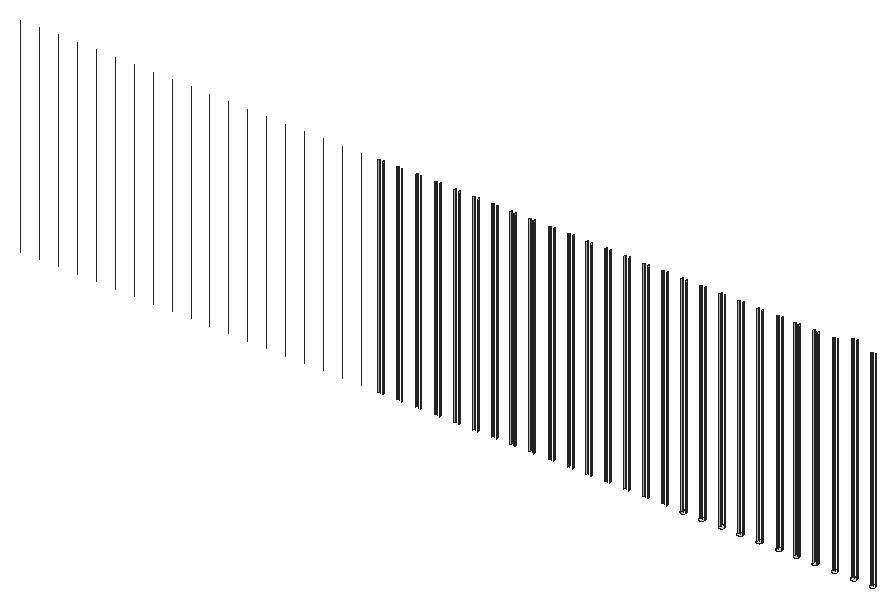
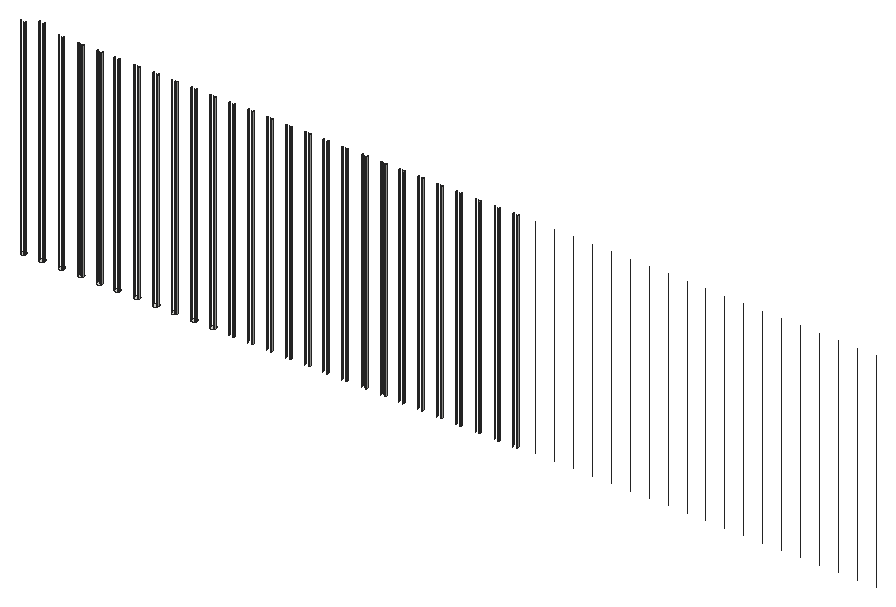
# SketchUp Ruby script. Lengths in inches.
U = 1.inch
M = Sketchup.active_model
def pt(a) = Geom::Point3d.new(a.map { |v| v * U })
def face(e, loops, mat)
  f = e.add_face(loops[0].map { |a| pt(a) })
  loops[1..].each { |l| e.add_face(l.map { |a| pt(a) }).erase! }
  f.material = f.back_material = mat if mat
  f
end
# faces: each face lists its corners as indices into pts; further lists are holes
def faces(e, pts, list, mat = nil) = list.each { |f| face(e, (f[0].is_a?(Array) ? f : [f]).map { |l| l.map { |i| pts[i] } }, mat) }
# xy, xz, yz: faces in a plane at the given z, y or x. An outline is a flat list of corners, or four numbers for a rectangle; further outlines are holes
def ring(l) = l.size == 4 ? [[l[0], l[1]], [l[2], l[1]], [l[2], l[3]], [l[0], l[3]]] : l.each_slice(2).to_a
def flat(e, list, mat, &to3) = list.each { |f| face(e, (f[0].is_a?(Array) ? f : [f]).map { |l| ring(l).map { |u, v| to3.(u, v) } }, mat) }
def xy(e, z, list, mat = nil) = flat(e, list, mat) { |x, y| [x, y, z] }
def xz(e, y, list, mat = nil) = flat(e, list, mat) { |x, z| [x, y, z] }
def yz(e, x, list, mat = nil) = flat(e, list, mat) { |y, z| [x, y, z] }
def lines(e, pts, list) = list.each { |a, b| e.add_line(pt(pts[a]), pt(pts[b])) }
# prism: a flat outline (further loops are holes) pulled along v
def prism(e, loops, v, mat = nil)
  f = face(e, loops, mat); d = Geom::Vector3d.new(v.map { |x| x * U })
  f.pushpull(f.normal.samedirection?(d) ? d.length : -d.length)
end
def box(e, o, s, mat = nil) = prism(e, [[o, [o[0] + s[0], o[1], o[2]], [o[0] + s[0], o[1] + s[1], o[2]], [o[0], o[1] + s[1], o[2]]]], [0, 0, s[2]], mat)
def at(x, y, z, deg = 0) = Geom::Transformation.translation(pt([x, y, z])) * Geom::Transformation.rotation(ORIGIN, Z_AXIS, deg.degrees)
def axes(o, x, y, z) = Geom::Transformation.new([*x, 0, *y, 0, *z, 0, *pt(o).to_a, 1])
def part(name) = M.definitions.add(name)
# library, detail: a bought-in or finely detailed component or shape, given as its bounding box
def library(name, o, s) = part(name).tap { |d| box(d.entities, o, s) }
def detail(e, o, s) = box(e.add_group.entities, o, s)
def put(e, d, t, mat = nil) = e.add_instance(d, t).tap { |i| i.material = mat if mat }
def group(e, t, mat = nil) = e.add_group.tap { |g| g.transformation = t; g.material = mat if mat }.entities
root = M.entities
xy(root,819.75,[[459.95,127.81,459.74,127.83,459.54,127.91,459.375,128.04,459.24,128.21,459.16,128.41,459.14,128.62,459.16,128.83,459.24,129.02,459.375,129.19,459.54,129.32,459.74,129.4,459.95,129.43,460.16,129.4,460.35,129.32,460.52,129.19,460.65,129.02,460.73,128.83,460.76,128.62,460.73,128.41,460.65,128.21,460.52,128.04,460.35,127.91,460.16,127.83],[465.76,127.81,465.55,127.83,465.35,127.91,465.1875,128.04,465.06,128.21,464.98,128.41,464.95,128.62,464.98,128.83,465.06,129.02,465.1875,129.19,465.35,129.32,465.55,129.4,465.76,129.43,465.97,129.4,466.17,129.32,466.34,129.19,466.46,129.02,466.55,128.83,466.57,128.62,466.55,128.41,466.46,128.21,466.34,128.04,466.17,127.91,465.97,127.83],[471.95,127.81,471.74,127.83,471.54,127.91,471.375,128.04,471.24,128.21,471.16,128.41,471.14,128.62,471.16,128.83,471.24,129.02,471.375,129.19,471.54,129.32,471.74,129.4,471.95,129.43,472.16,129.4,472.35,129.32,472.52,129.19,472.65,129.02,472.73,128.83,472.76,128.62,472.73,128.41,472.65,128.21,472.52,128.04,472.35,127.91,472.16,127.83],[477.76,127.81,477.55,127.83,477.35,127.91,477.1875,128.04,477.06,128.21,476.98,128.41,476.95,128.62,476.98,128.83,477.06,129.02,477.1875,129.19,477.35,129.32,477.55,129.4,477.76,129.43,477.97,129.4,478.17,129.32,478.34,129.19,478.46,129.02,478.55,128.83,478.57,128.62,478.55,128.41,478.46,128.21,478.34,128.04,478.17,127.91,477.97,127.83],[483.76,127.81,483.55,127.83,483.35,127.91,483.1875,128.04,483.06,128.21,482.98,128.41,482.95,128.62,482.98,128.83,483.06,129.02,483.1875,129.19,483.35,129.32,483.55,129.4,483.76,129.43,483.97,129.4,484.17,129.32,484.34,129.19,484.46,129.02,484.55,128.83,484.57,128.62,484.55,128.41,484.46,128.21,484.34,128.04,484.17,127.91,483.97,127.83],
  [489.89,127.81,489.68,127.83,489.48,127.91,489.3125,128.04,489.18,128.21,489.1,128.41,489.07,128.62,489.1,128.83,489.18,129.02,489.3125,129.19,489.48,129.32,489.68,129.4,489.89,129.43,490.1,129.4,490.29,129.32,490.46,129.19,490.59,129.02,490.67,128.83,490.7,128.62,490.67,128.41,490.59,128.21,490.46,128.04,490.29,127.91,490.1,127.83],[495.39,127.81,495.18,127.83,494.98,127.91,494.8125,128.04,494.68,128.21,494.6,128.41,494.57,128.62,494.6,128.83,494.68,129.02,494.8125,129.19,494.98,129.32,495.18,129.4,495.39,129.43,495.6,129.4,495.79,129.32,495.96,129.19,496.09,129.02,496.17,128.83,496.2,128.62,496.17,128.41,496.09,128.21,495.96,128.04,495.79,127.91,495.6,127.83],[501.32,127.81,501.11,127.83,500.92,127.91,500.75,128.04,500.62,128.21,500.54,128.41,500.51,128.62,500.54,128.83,500.62,129.02,500.75,129.19,500.92,129.32,501.11,129.4,501.32,129.43,501.53,129.4,501.73,129.32,501.9,129.19,502.03,129.02,502.11,128.83,502.14,128.62,502.11,128.41,502.03,128.21,501.9,128.04,501.73,127.91,501.53,127.83],[507.39,127.81,507.18,127.83,506.98,127.91,506.8125,128.04,506.68,128.21,506.6,128.41,506.57,128.62,506.6,128.83,506.68,129.02,506.8125,129.19,506.98,129.32,507.18,129.4,507.39,129.43,507.6,129.4,507.79,129.32,507.96,129.19,508.09,129.02,508.17,128.83,508.2,128.62,508.17,128.41,508.09,128.21,507.96,128.04,507.79,127.91,507.6,127.83],[513.45,127.81,513.24,127.83,513.04,127.91,512.875,128.04,512.74,128.21,512.66,128.41,512.64,128.62,512.66,128.83,512.74,129.02,512.875,129.19,513.04,129.32,513.24,129.4,513.45,129.43,513.66,129.4,513.85,129.32,514.02,129.19,514.15,129.02,514.23,128.83,514.26,128.62,514.23,128.41,514.15,128.21,514.02,128.04,513.85,127.91,513.66,127.83],
  [519.32,127.81,519.11,127.83,518.92,127.91,518.75,128.04,518.62,128.21,518.54,128.41,518.51,128.62,518.54,128.83,518.62,129.02,518.75,129.19,518.92,129.32,519.11,129.4,519.32,129.43,519.53,129.4,519.73,129.32,519.9,129.19,520.03,129.02,520.11,128.83,520.14,128.62,520.11,128.41,520.03,128.21,519.9,128.04,519.73,127.91,519.53,127.83]])
p = [[364.23,128.83,819.75],[364.2,128.62,819.75],[364.2,128.62,884.89],[364.23,128.83,884.89],[365.82,128.62,819.75],[365.8,128.83,819.75],
  [365.8,128.83,884.89],[365.82,128.62,884.89],[369.98,128.83,819.75],[369.95,128.62,819.75],[369.95,128.62,884.89],[369.98,128.83,884.89],
  [371.57,128.62,819.75],[371.55,128.83,819.75],[371.55,128.83,884.89],[371.57,128.62,884.89],[375.91,128.83,819.75],[375.89,128.62,819.75],
  [375.89,128.62,884.89],[375.91,128.83,884.89],[377.51,128.62,819.75],[377.48,128.83,819.75],[377.48,128.83,884.89],[377.51,128.62,884.89],
  [381.98,128.83,819.75],[381.95,128.62,819.75],[381.95,128.62,884.89],[381.98,128.83,884.89],[383.57,128.62,819.75],[383.55,128.83,819.75],
  [383.55,128.83,884.89],[383.57,128.62,884.89],[388.04,128.83,819.75],[388.01,128.62,819.75],[388.01,128.62,884.89],[388.04,128.83,884.89],
  [389.64,128.62,819.75],[389.61,128.83,819.75],[389.61,128.83,884.89],[389.64,128.62,884.89],[393.98,128.83,819.75],[393.95,128.62,819.75],
  [393.95,128.62,884.89],[393.98,128.83,884.89],[395.57,128.62,819.75],[395.55,128.83,819.75],[395.55,128.83,884.89],[395.57,128.62,884.89],
  [399.79,128.83,819.75],[399.76,128.62,819.75],[399.76,128.62,884.89],[399.79,128.83,884.89],[401.39,128.62,819.75],[401.36,128.83,819.75],
  [401.36,128.83,884.89],[401.39,128.62,884.89],[405.6,128.83,819.75],[405.57,128.62,819.75],[405.57,128.62,884.89],[405.6,128.83,884.89],
  [407.2,128.62,819.75],[407.17,128.83,819.75],[407.17,128.83,884.89],[407.2,128.62,884.89],[411.54,128.83,819.75],[411.51,128.62,819.75],
  [411.51,128.62,884.89],[411.54,128.83,884.89],[413.14,128.62,819.75],[413.11,128.83,819.75],[413.11,128.83,884.89],[413.14,128.62,884.89],
  [417.66,128.83,819.75],[417.64,128.62,819.75],[417.64,128.62,884.89],[417.66,128.83,884.89],[419.26,128.62,819.75],[419.23,128.83,819.75],
  [419.23,128.83,884.89],[419.26,128.62,884.89],[423.6,128.83,819.75],[423.57,128.62,819.75],[423.57,128.62,884.89],[423.6,128.83,884.89],
  [425.2,128.62,819.75],[425.17,128.83,819.75],[425.17,128.83,884.89],[425.2,128.62,884.89],[429.41,128.83,819.75],[429.39,128.62,819.75],
  [429.39,128.62,884.89],[429.41,128.83,884.89],[431.01,128.62,819.75],[430.98,128.83,819.75],[430.98,128.83,884.89],[431.01,128.62,884.89],
  [435.23,128.83,819.75],[435.2,128.62,819.75],[435.2,128.62,884.89],[435.23,128.83,884.89],[436.82,128.62,819.75],[436.8,128.83,819.75],
  [436.8,128.83,884.89],[436.82,128.62,884.89],[441.23,128.83,819.75],[441.2,128.62,819.75],[441.2,128.62,884.89],[441.23,128.83,884.89],
  [442.82,128.62,819.75],[442.8,128.83,819.75],[442.8,128.83,884.89],[442.82,128.62,884.89],[447.29,128.83,819.75],[447.26,128.62,819.75],
  [447.26,128.62,884.89],[447.29,128.83,884.89],[448.89,128.62,819.75],[448.86,128.83,819.75],[448.86,128.83,884.89],[448.89,128.62,884.89],
  [453.1,128.83,819.75],[453.07,128.62,819.75],[453.07,128.62,884.89],[453.1,128.83,884.89],[454.7,128.62,819.75],[454.67,128.83,819.75],
  [454.67,128.83,884.89],[454.7,128.62,884.89],[459.16,128.83,819.75],[459.14,128.62,819.75],[459.14,128.62,884.89],[459.16,128.83,884.89],
  [460.76,128.62,819.75],[460.73,128.83,819.75],[460.73,128.83,884.89],[460.76,128.62,884.89],[464.98,128.83,819.75],[464.95,128.62,819.75],
  [464.95,128.62,884.89],[464.98,128.83,884.89],[466.57,128.62,819.75],[466.55,128.83,819.75],[466.55,128.83,884.89],[466.57,128.62,884.89],
  [471.16,128.83,819.75],[471.14,128.62,819.75],[471.14,128.62,884.89],[471.16,128.83,884.89],[472.76,128.62,819.75],[472.73,128.83,819.75],
  [472.73,128.83,884.89],[472.76,128.62,884.89],[476.98,128.83,819.75],[476.95,128.62,819.75],[476.95,128.62,884.89],[476.98,128.83,884.89],
  [478.57,128.62,819.75],[478.55,128.83,819.75],[478.55,128.83,884.89],[478.57,128.62,884.89],[482.98,128.83,819.75],[482.95,128.62,819.75],
  [482.95,128.62,884.89],[482.98,128.83,884.89],[484.57,128.62,819.75],[484.55,128.83,819.75],[484.55,128.83,884.89],[484.57,128.62,884.89],
  [489.1,128.83,819.75],[489.07,128.62,819.75],[489.07,128.62,884.89],[489.1,128.83,884.89],[490.7,128.62,819.75],[490.67,128.83,819.75],
  [490.67,128.83,884.89],[490.7,128.62,884.89],[494.6,128.83,819.75],[494.57,128.62,819.75],[494.57,128.62,884.89],[494.6,128.83,884.89],
  [496.2,128.62,819.75],[496.17,128.83,819.75],[496.17,128.83,884.89],[496.2,128.62,884.89],[500.54,128.83,819.75],[500.51,128.62,819.75],
  [500.51,128.62,884.89],[500.54,128.83,884.89],[502.14,128.62,819.75],[502.11,128.83,819.75],[502.11,128.83,884.89],[502.14,128.62,884.89],
  [506.6,128.83,819.75],[506.57,128.62,819.75],[506.57,128.62,884.89],[506.6,128.83,884.89],[508.2,128.62,819.75],[508.17,128.83,819.75],
  [508.17,128.83,884.89],[508.2,128.62,884.89],[512.66,128.83,819.75],[512.64,128.62,819.75],[512.64,128.62,886.75],[512.66,128.83,886.75],
  [514.26,128.62,819.75],[514.23,128.83,819.75],[514.23,128.83,886.75],[514.26,128.62,886.75],[518.54,128.83,819.75],[518.51,128.62,819.75],
  [518.51,128.62,884.89],[518.54,128.83,884.89],[520.14,128.62,819.75],[520.11,128.83,819.75],[520.11,128.83,884.89],[520.14,128.62,884.89],
  [364.31,129.02,819.75],[364.31,129.02,884.89],[365.71,129.02,819.75],[365.71,129.02,884.89],[370.06,129.02,819.75],[370.06,129.02,884.89],
  [371.46,129.02,819.75],[371.46,129.02,884.89],[375.99,129.02,819.75],[375.99,129.02,884.89],[377.4,129.02,819.75],[377.4,129.02,884.89],
  [382.06,129.02,819.75],[382.06,129.02,884.89],[383.46,129.02,819.75],[383.46,129.02,884.89],[388.12,129.02,819.75],[388.12,129.02,884.89],
  [389.53,129.02,819.75],[389.53,129.02,884.89],[394.06,129.02,819.75],[394.06,129.02,884.89],[395.46,129.02,819.75],[395.46,129.02,884.89],
  [399.87,129.02,819.75],[399.87,129.02,884.89],[401.28,129.02,819.75],[401.28,129.02,884.89],[405.68,129.02,819.75],[405.68,129.02,884.89],
  [407.09,129.02,819.75],[407.09,129.02,884.89],[411.62,129.02,819.75],[411.62,129.02,884.89],[413.03,129.02,819.75],[413.03,129.02,884.89],
  [417.74,129.02,819.75],[417.74,129.02,884.89],[419.15,129.02,819.75],[419.15,129.02,884.89],[423.68,129.02,819.75],[423.68,129.02,884.89],
  [425.09,129.02,819.75],[425.09,129.02,884.89],[429.49,129.02,819.75],[429.49,129.02,884.89],[430.9,129.02,819.75],[430.9,129.02,884.89],
  [435.31,129.02,819.75],[435.31,129.02,884.89],[436.71,129.02,819.75],[436.71,129.02,884.89],[441.31,129.02,819.75],[441.31,129.02,884.89],
  [442.71,129.02,819.75],[442.71,129.02,884.89],[447.37,129.02,819.75],[447.37,129.02,884.89],[448.78,129.02,819.75],[448.78,129.02,884.89],
  [453.18,129.02,819.75],[453.18,129.02,884.89],[454.59,129.02,819.75],[454.59,129.02,884.89],[459.24,129.02,819.75],[459.24,129.02,884.89],
  [460.65,129.02,819.75],[460.65,129.02,884.89],[465.06,129.02,819.75],[465.06,129.02,884.89],[466.46,129.02,819.75],[466.46,129.02,884.89],
  [471.24,129.02,819.75],[471.24,129.02,884.89],[472.65,129.02,819.75],[472.65,129.02,884.89],[477.06,129.02,819.75],[477.06,129.02,884.89],
  [478.46,129.02,819.75],[478.46,129.02,884.89],[483.06,129.02,819.75],[483.06,129.02,884.89],[484.46,129.02,819.75],[484.46,129.02,884.89],
  [489.18,129.02,819.75],[489.18,129.02,884.89],[490.59,129.02,819.75],[490.59,129.02,884.89],[494.68,129.02,819.75],[494.68,129.02,884.89],
  [496.09,129.02,819.75],[496.09,129.02,884.89],[500.62,129.02,819.75],[500.62,129.02,884.89],[502.03,129.02,819.75],[502.03,129.02,884.89],
  [506.68,129.02,819.75],[506.68,129.02,884.89],[508.09,129.02,819.75],[508.09,129.02,884.89],[512.74,129.02,819.75],[512.74,129.02,886.75],
  [514.15,129.02,819.75],[514.15,129.02,886.75],[518.62,129.02,819.75],[518.62,129.02,884.89],[520.03,129.02,819.75],[520.03,129.02,884.89],
  [364.4375,129.19,819.75],[364.4375,129.19,884.89],[365.59,129.19,819.75],[365.59,129.19,884.89],[370.1875,129.19,819.75],[370.1875,129.19,884.89],
  [376.125,129.19,819.75],[376.125,129.19,884.89],[377.27,129.19,819.75],[377.27,129.19,884.89],[382.1875,129.19,819.75],[382.1875,129.19,884.89],
  [383.34,129.19,819.75],[383.34,129.19,884.89],[388.25,129.19,819.75],[388.25,129.19,884.89],[389.4,129.19,819.75],[389.4,129.19,884.89],
  [394.1875,129.19,819.75],[394.1875,129.19,884.89],[395.34,129.19,819.75],[395.34,129.19,884.89],[400,129.19,819.75],[400,129.19,884.89],
  [401.15,129.19,819.75],[401.15,129.19,884.89],[405.8125,129.19,819.75],[405.8125,129.19,884.89],[406.96,129.19,819.75],[406.96,129.19,884.89],
  [411.75,129.19,819.75],[411.75,129.19,884.89],[412.9,129.19,819.75],[412.9,129.19,884.89],[417.875,129.19,819.75],[417.875,129.19,884.89],
  [419.02,129.19,819.75],[419.02,129.19,884.89],[423.8125,129.19,819.75],[423.8125,129.19,884.89],[424.96,129.19,819.75],[424.96,129.19,884.89],
  [429.625,129.19,819.75],[429.625,129.19,884.89],[430.77,129.19,819.75],[430.77,129.19,884.89],[435.4375,129.19,819.75],[435.4375,129.19,884.89],
  [436.59,129.19,819.75],[436.59,129.19,884.89],[441.4375,129.19,819.75],[441.4375,129.19,884.89],[442.59,129.19,819.75],[442.59,129.19,884.89],
  [447.5,129.19,819.75],[447.5,129.19,884.89],[448.65,129.19,819.75],[448.65,129.19,884.89],[453.3125,129.19,819.75],[453.3125,129.19,884.89],
  [454.46,129.19,819.75],[454.46,129.19,884.89],[459.375,129.19,819.75],[459.375,129.19,884.89],[460.52,129.19,819.75],[460.52,129.19,884.89],
  [465.1875,129.19,819.75],[465.1875,129.19,884.89],[466.34,129.19,819.75],[466.34,129.19,884.89],[471.375,129.19,819.75],[471.375,129.19,884.89],
  [472.52,129.19,819.75],[472.52,129.19,884.89],[477.1875,129.19,819.75],[477.1875,129.19,884.89],[478.34,129.19,819.75],[478.34,129.19,884.89],
  [483.1875,129.19,819.75],[483.1875,129.19,884.89],[484.34,129.19,819.75],[484.34,129.19,884.89],[489.3125,129.19,819.75],[489.3125,129.19,884.89],
  [490.46,129.19,819.75],[490.46,129.19,884.89],[494.8125,129.19,819.75],[494.8125,129.19,884.89],[495.96,129.19,819.75],[495.96,129.19,884.89],
  [500.75,129.19,819.75],[500.75,129.19,884.89],[501.9,129.19,819.75],[501.9,129.19,884.89],[506.8125,129.19,819.75],[506.8125,129.19,884.89],
  [507.96,129.19,819.75],[507.96,129.19,884.89],[512.875,129.19,819.75],[512.875,129.19,886.75],[514.02,129.19,819.75],[514.02,129.19,886.75],
  [518.75,129.19,819.75],[518.75,129.19,884.89],[519.9,129.19,819.75],[519.9,129.19,884.89],[519.29,128.62,884.89],[519.29,128.62,819.75],
  [513.35,128.62,884.89],[513.35,128.62,819.75],[507.41,128.62,884.89],[507.41,128.62,819.75],[501.47,128.62,884.89],[501.47,128.62,819.75],
  [495.54,128.62,884.89],[495.54,128.62,819.75],[489.6,128.62,884.89],[489.6,128.62,819.75],[483.66,128.62,884.89],[483.66,128.62,819.75],
  [477.72,128.62,884.89],[477.72,128.62,819.75],[471.79,128.62,884.89],[471.79,128.62,819.75],[465.85,128.62,884.89],[465.85,128.62,819.75],
  [459.91,128.62,884.89],[459.91,128.62,819.75],[453.97,128.62,884.89],[453.97,128.62,819.75],[448.04,128.62,884.89],[448.04,128.62,819.75],
  [442.1,128.62,884.89],[442.1,128.62,819.75],[436.16,128.62,884.89],[436.16,128.62,819.75],[430.22,128.62,884.89],[430.22,128.62,819.75],
  [424.29,128.62,884.89],[424.29,128.62,819.75],[418.35,128.62,884.89],[418.35,128.62,819.75],[412.41,128.62,884.89],[412.41,128.62,819.75],
  [406.47,128.62,884.89],[406.47,128.62,819.75],[400.54,128.62,884.89],[400.54,128.62,819.75],[394.6,128.62,884.89],[394.6,128.62,819.75],
  [388.66,128.62,884.89],[388.66,128.62,819.75],[382.72,128.62,884.89],[382.72,128.62,819.75],[376.79,128.62,884.89],[376.79,128.62,819.75],
  [370.85,128.62,884.89],[370.85,128.62,819.75],[364.91,128.62,884.89],[364.91,128.62,819.75],[358.97,128.62,884.89],[358.97,128.62,819.75],
  [353.04,128.62,884.89],[353.04,128.62,819.75],[347.1,128.62,884.89],[347.1,128.62,819.75],[341.16,128.62,884.89],[341.16,128.62,819.75],
  [335.22,128.62,884.89],[335.22,128.62,819.75],[329.29,128.62,884.89],[329.29,128.62,819.75],[323.35,128.62,884.89],[323.35,128.62,819.75],
  [317.41,128.62,884.89],[317.41,128.62,819.75],[311.47,128.62,884.89],[311.47,128.62,819.75],[305.54,128.62,884.89],[305.54,128.62,819.75],
  [299.6,128.62,884.89],[299.6,128.62,819.75],[293.66,128.62,884.89],[293.66,128.62,819.75],[287.72,128.62,884.89],[287.72,128.62,819.75],
  [281.79,128.62,884.89],[281.79,128.62,819.75],[275.85,128.62,884.89],[275.85,128.62,819.75],[269.91,128.62,884.89],[269.91,128.62,819.75],
  [263.97,128.62,884.89],[263.97,128.62,819.75],[258.04,128.62,884.89],[258.04,128.62,819.75],[252.1,128.62,884.89],[252.1,128.62,819.75]]
faces(root,p,[[0,1,2,3],[4,5,6,7],[8,9,10,11],[12,13,14,15],[16,17,18,19],[20,21,22,23],[24,25,26,27],[28,29,30,31],
  [32,33,34,35],[36,37,38,39],[40,41,42,43],[44,45,46,47],[48,49,50,51],[52,53,54,55],[56,57,58,59],[60,61,62,63],
  [64,65,66,67],[68,69,70,71],[72,73,74,75],[76,77,78,79],[80,81,82,83],[84,85,86,87],[88,89,90,91],[92,93,94,95],
  [96,97,98,99],[100,101,102,103],[104,105,106,107],[108,109,110,111],[112,113,114,115],[116,117,118,119],[120,121,122,123],[124,125,126,127],
  [128,129,130,131],[132,133,134,135],[136,137,138,139],[140,141,142,143],[144,145,146,147],[148,149,150,151],[152,153,154,155],[156,157,158,159],
  [160,161,162,163],[164,165,166,167],[168,169,170,171],[172,173,174,175],[176,177,178,179],[180,181,182,183],[184,185,186,187],[188,189,190,191],
  [192,193,194,195],[196,197,198,199],[200,201,202,203],[204,205,206,207],[208,209,210,211],[212,213,214,215],[216,0,3,217],[5,218,219,6],
  [220,8,11,221],[13,222,223,14],[224,16,19,225],[21,226,227,22],[228,24,27,229],[29,230,231,30],[232,32,35,233],[37,234,235,38],
  [236,40,43,237],[45,238,239,46],[240,48,51,241],[53,242,243,54],[244,56,59,245],[61,246,247,62],[248,64,67,249],[69,250,251,70],
  [252,72,75,253],[77,254,255,78],[256,80,83,257],[85,258,259,86],[260,88,91,261],[93,262,263,94],[264,96,99,265],[101,266,267,102],
  [268,104,107,269],[109,270,271,110],[272,112,115,273],[117,274,275,118],[276,120,123,277],[125,278,279,126],[280,128,131,281],[133,282,283,134],
  [284,136,139,285],[141,286,287,142],[288,144,147,289],[149,290,291,150],[292,152,155,293],[157,294,295,158],[296,160,163,297],[165,298,299,166],
  [300,168,171,301],[173,302,303,174],[304,176,179,305],[181,306,307,182],[308,184,187,309],[189,310,311,190],[312,192,195,313],[197,314,315,198],
  [316,200,203,317],[205,318,319,206],[320,208,211,321],[213,322,323,214],[324,216,217,325],[218,326,327,219],[328,220,221,329],[330,224,225,331],
  [226,332,333,227],[334,228,229,335],[230,336,337,231],[338,232,233,339],[234,340,341,235],[342,236,237,343],[238,344,345,239],[346,240,241,347],
  [242,348,349,243],[350,244,245,351],[246,352,353,247],[354,248,249,355],[250,356,357,251],[358,252,253,359],[254,360,361,255],[362,256,257,363],
  [258,364,365,259],[366,260,261,367],[262,368,369,263],[370,264,265,371],[266,372,373,267],[374,268,269,375],[270,376,377,271],[378,272,273,379],
  [274,380,381,275],[382,276,277,383],[278,384,385,279],[386,280,281,387],[282,388,389,283],[390,284,285,391],[286,392,393,287],[394,288,289,395],
  [290,396,397,291],[398,292,293,399],[294,400,401,295],[402,296,297,403],[298,404,405,299],[406,300,301,407],[302,408,409,303],[410,304,305,411],
  [306,412,413,307],[414,308,309,415],[310,416,417,311],[418,312,313,419],[314,420,421,315],[422,316,317,423],[318,424,425,319],[426,320,321,427],
  [322,428,429,323]])
lines(root,p,[[430,431],[432,433],[434,435],[436,437],[438,439],[440,441],[442,443],[444,445],[446,447],[448,449],[450,451],[452,453],
  [454,455],[456,457],[458,459],[460,461],[462,463],[464,465],[466,467],[468,469],[470,471],[472,473],[474,475],[476,477],
  [478,479],[480,481],[482,483],[484,485],[486,487],[488,489],[490,491],[492,493],[494,495],[496,497],[498,499],[500,501],
  [502,503],[504,505],[506,507],[508,509],[510,511],[512,513],[514,515],[516,517],[518,519],[520,521]])
